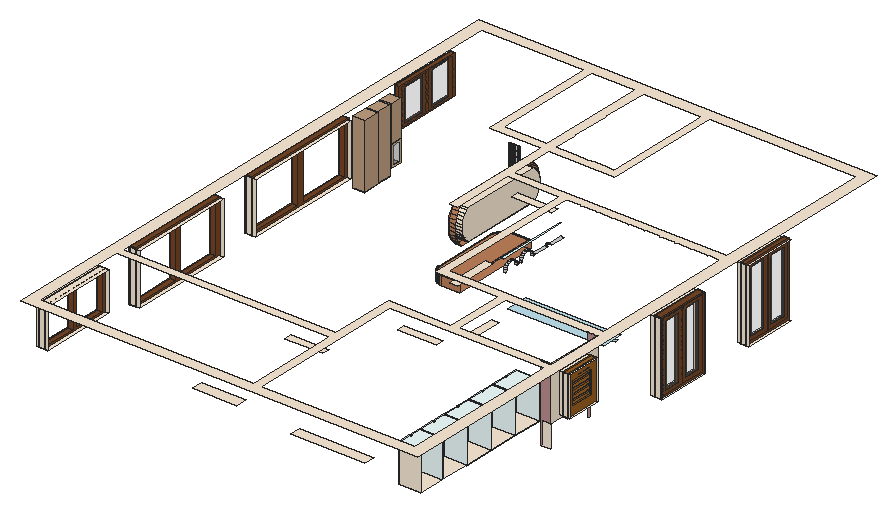
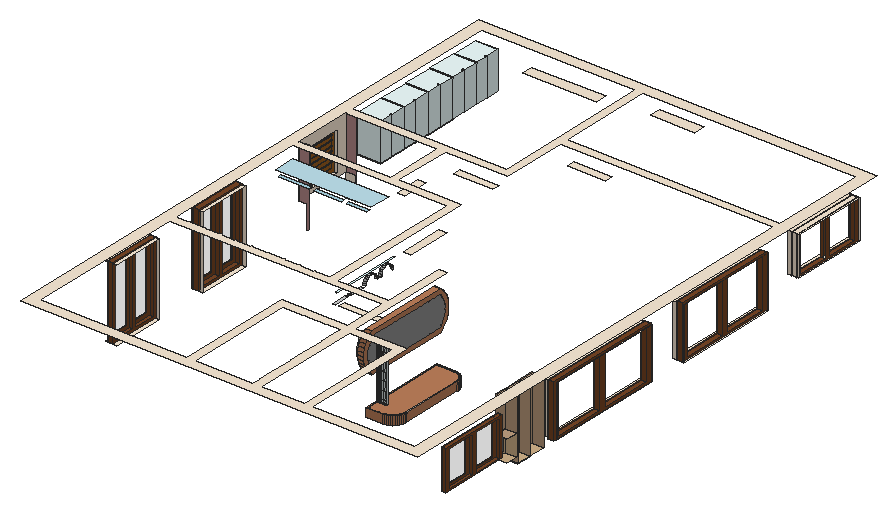
# SketchUp Ruby script. Lengths in inches.
U = 1.inch
M = Sketchup.active_model
def pt(a) = Geom::Point3d.new(a.map { |v| v * U })
def face(e, loops, mat)
  f = e.add_face(loops[0].map { |a| pt(a) })
  loops[1..].each { |l| e.add_face(l.map { |a| pt(a) }).erase! }
  f.material = f.back_material = mat if mat
  f
end
# faces: each face lists its corners as indices into pts; further lists are holes
def faces(e, pts, list, mat = nil) = list.each { |f| face(e, (f[0].is_a?(Array) ? f : [f]).map { |l| l.map { |i| pts[i] } }, mat) }
# xy, xz, yz: faces in a plane at the given z, y or x. An outline is a flat list of corners, or four numbers for a rectangle; further outlines are holes
def ring(l) = l.size == 4 ? [[l[0], l[1]], [l[2], l[1]], [l[2], l[3]], [l[0], l[3]]] : l.each_slice(2).to_a
def flat(e, list, mat, &to3) = list.each { |f| face(e, (f[0].is_a?(Array) ? f : [f]).map { |l| ring(l).map { |u, v| to3.(u, v) } }, mat) }
def xy(e, z, list, mat = nil) = flat(e, list, mat) { |x, y| [x, y, z] }
def xz(e, y, list, mat = nil) = flat(e, list, mat) { |x, z| [x, y, z] }
def yz(e, x, list, mat = nil) = flat(e, list, mat) { |y, z| [x, y, z] }
def lines(e, pts, list) = list.each { |a, b| e.add_line(pt(pts[a]), pt(pts[b])) }
# prism: a flat outline (further loops are holes) pulled along v
def prism(e, loops, v, mat = nil)
  f = face(e, loops, mat); d = Geom::Vector3d.new(v.map { |x| x * U })
  f.pushpull(f.normal.samedirection?(d) ? d.length : -d.length)
end
def box(e, o, s, mat = nil) = prism(e, [[o, [o[0] + s[0], o[1], o[2]], [o[0] + s[0], o[1] + s[1], o[2]], [o[0], o[1] + s[1], o[2]]]], [0, 0, s[2]], mat)
def at(x, y, z, deg = 0) = Geom::Transformation.translation(pt([x, y, z])) * Geom::Transformation.rotation(ORIGIN, Z_AXIS, deg.degrees)
def axes(o, x, y, z) = Geom::Transformation.new([*x, 0, *y, 0, *z, 0, *pt(o).to_a, 1])
def part(name) = M.definitions.add(name)
# library, detail: a bought-in or finely detailed component or shape, given as its bounding box
def library(name, o, s) = part(name).tap { |d| box(d.entities, o, s) }
def detail(e, o, s) = box(e.add_group.entities, o, s)
def put(e, d, t, mat = nil) = e.add_instance(d, t).tap { |i| i.material = mat if mat }
def group(e, t, mat = nil) = e.add_group.tap { |g| g.transformation = t; g.material = mat if mat }.entities
root = M.entities
M.materials.add("Plywood A 50cm\#1").color = [191, 159, 129]
M.materials.add("Wood EXN").color = [155, 95, 32]
M.materials.add("[0028_AntiqueWhite]").color = [250, 235, 215]
M.materials.add("[0035_Tan]").color = [210, 180, 140]
M.materials.add("[0090_LightCyan]").color = [224, 255, 255]
M.materials.add("[0092_Azure]").color = [240, 255, 255]
M.materials.add("[0095_LightBlue]").color = [173, 216, 230]
M.materials.add("[0100_SteelBlue]").color = [70, 130, 180]
M.materials.add("[0119_RosyBrown]").color = [188, 143, 143]
M.materials.add("[Carrera Marble]").color = [207, 207, 207]
M.materials.add("[Color M04]").color = [142, 142, 142]
M.materials.add("[Steel]").color = [192, 228, 240]
M.materials.add("[Translucent Glass Gray]").color = [128, 128, 128]
M.materials["[Translucent Glass Gray]"].alpha = 0.5
M.materials.add("[Translucent Glass Gray]1").color = [132, 132, 132]
M.materials["[Translucent Glass Gray]1"].alpha = 0.25
M.materials.add("[Wallpaper Dog Bone]").color = [213, 224, 224]
M.materials.add("[Wood Veneer 01]").color = [120, 70, 37]
M.materials.add("[Wood Veneer 02]").color = [190, 128, 91]
c1 = part("Group\#38")
prism(c1.entities,[[[0,1.97,1.57],[0,0.24,0.19],[0,0.22,0.17],[0,0.2,0.14],[0,0.19,0.11],[0,0.2,0.08],[0,0.2,0.05],[0,0.22,0.02],[0,0.24,0],[0,0.27,-0.02],[0,0.3,-0.03],[0,0.34,-0.03],[0,0.37,-0.02],[0,0.39,0],[0,2.36,1.57]]],[-67.04,0,0])
c2 = part("Wood+Window")
g1 = group(c2.entities,at(47.24,0,19.69),"Wood EXN")
g2 = group(g1,at(-47.24,5.91,0))
xy(g2,-19.69,[[0,-5.91,27.56,0]])
xy(g2,-17.72,[[1.97,-3.9375,25.59,0]])
xy(g2,-15.75,[[3.9375,-5.91,23.62,-4.92],[3.9375,-4.92,23.62,-3.9375]])
xy(g2,-3.9375,[[3.9375,-5.91,23.62,-4.92],[3.9375,-4.92,23.62,-3.9375]])
xy(g2,-1.97,[[1.97,-3.9375,25.59,0]])
xy(g2,0,[[0,-5.91,27.56,0]])
xz(g2,-5.91,[[[0,-19.69,27.56,0],[3.9375,-15.75,23.62,-3.9375]]])
xz(g2,-3.9375,[[[1.97,-17.72,25.59,-1.97],[3.9375,-15.75,23.62,-3.9375]]])
xz(g2,0,[[[0,-19.69,27.56,0],[1.97,-17.72,25.59,-1.97]]])
yz(g2,0,[[-5.91,-19.69,0,0]])
yz(g2,1.97,[[-3.9375,-17.72,0,-1.97]])
yz(g2,3.9375,[[-5.91,-15.75,-4.92,-3.9375],[-4.92,-15.75,-3.9375,-3.9375]])
yz(g2,23.62,[[-5.91,-15.75,-4.92,-3.9375],[-4.92,-15.75,-3.9375,-3.9375]])
yz(g2,25.59,[[-3.9375,-17.72,0,-1.97]])
yz(g2,27.56,[[-5.91,-19.69,0,0]])
g3 = group(g1,at(-20.98,5.88,-0.4))
put(g3,c1,axes([-24.3,0,-14.09],[-0.35238,0,0],[0,0,-1.2344],[0,-1,0]))
put(g3,c1,axes([-24.3,0,-11.66],[-0.35238,0,0],[0,0,-1.2344],[0,-1,0]))
put(g3,c1,axes([-24.3,0,-9.23],[-0.35238,0,0],[0,0,-1.2344],[0,-1,0]))
put(g3,c1,axes([-24.3,0,-6.8],[-0.35238,0,0],[0,0,-1.2344],[0,-1,0]))
put(g3,c1,axes([-24.3,0,-4.375],[-0.35238,0,0],[0,0,-1.2344],[0,-1,0]))
put(g3,c1,axes([-24.3,0,-1.94],[-0.35238,0,0],[0,0,-1.2344],[0,-1,0]))
c3 = part("Group\#31")
xy(c3.entities,0,[[0,0,19.69,1.18]],"[Wood Veneer 01]")
xy(c3.entities,2.76,[[2.76,0,16.93,1.18]],"[Wood Veneer 01]")
xy(c3.entities,60.24,[[2.76,0,16.93,1.18]],"[Wood Veneer 01]")
xy(c3.entities,62.99,[[0,0,19.69,1.18]],"[Wood Veneer 01]")
xz(c3.entities,0,[[2.76,2.76,16.93,60.24]],"[Translucent Glass Gray]1")
xz(c3.entities,0,[[[0,0,19.69,62.99],[2.76,2.76,16.93,60.24]]],"[Wood Veneer 01]")
xz(c3.entities,1.18,[[[0,0,19.69,62.99],[2.76,2.76,16.93,60.24]]],"[Wood Veneer 01]")
yz(c3.entities,0,[[0,0,1.18,62.99]],"[Wood Veneer 01]")
yz(c3.entities,2.76,[[0,2.76,1.18,60.24]],"[Wood Veneer 01]")
yz(c3.entities,16.93,[[0,2.76,1.18,60.24]],"[Wood Veneer 01]")
yz(c3.entities,19.69,[[0,0,1.18,62.99]],"[Wood Veneer 01]")
c4 = part("Group\#45")
prism(c4.entities,[[[0,0,66.93],[0,0,0],[45.28,0,0],[45.28,0,66.93]],[[43.31,0,1.97],[23.62,0,1.97],[23.62,0,64.96],[43.31,0,64.96]],[[21.65,0,64.96],[21.65,0,1.97],[1.97,0,1.97],[1.97,0,64.96]]],[0,5.91,0],"[Wood Veneer 01]")
c5 = part("pintu 2")
put(c5.entities,c3,axes([-252.08,-272.33,20.79],[0,0.96078,0],[-0.7,0,0],[0,0,0.89]))
put(c5.entities,c4,axes([-252.08,-295.03,19.04],[0,0.96078,0],[-0.7,0,0],[0,0,0.89]))
put(c5.entities,c3,axes([-252.08,-293.14,20.79],[0,0.96078,0],[-0.7,0,0],[0,0,0.89]))
put(c5.entities,c3,axes([-251.13,-360.52,20.79],[0,0.95802,0],[-0.861,0,0],[0,0,0.89]))
put(c5.entities,c4,axes([-251.13,-383.15,19.04],[0,0.95802,0],[-0.861,0,0],[0,0,0.89]))
put(c5.entities,c3,axes([-251.13,-381.27,20.79],[0,0.95802,0],[-0.861,0,0],[0,0,0.89]))
put(c5.entities,c3,axes([-569.23,-250.27,47.16],[0,1.26545,0],[-0.63714,0,0],[0,0,0.47766]))
put(c5.entities,c4,axes([-569.23,-252.76,46.22],[0,1.26545,0],[-0.63714,0,0],[0,0,0.47766]))
put(c5.entities,c3,axes([-569.23,-222.87,47.16],[0,1.26545,0],[-0.63714,0,0],[0,0,0.47766]))
g4 = group(c5.entities,at(-568.41,-522.34,36.16))
prism(g4,[[[0,0,42.82],[0,0,0],[0,85.875,0],[0,85.875,42.82]],[[0,82.14,1.26],[0,44.8,1.26],[0,44.8,41.56],[0,82.14,41.56]],[[0,41.07,41.56],[0,41.07,1.26],[0,3.73,1.26],[0,3.73,41.56]]],[-4.84,0,0],"[Wood Veneer 01]")
xy(g4,10.99,[[-4.61,-90.31,0,-63.41],[-4.61,-60.72,0,-33.82]],"[Wood Veneer 01]")
xz(g4,-90.31,[[-4.61,10.99,0,40.82]],"[Wood Veneer 01]")
xz(g4,-63.41,[[-4.61,10.99,0,40.82]],"[Wood Veneer 01]")
xz(g4,-33.82,[[-4.61,10.99,0,40.82]],"[Wood Veneer 01]")
yz(g4,-4.61,[[[-93,10.0625,-31.125,41.75],[-90.31,10.99,-63.41,40.82],[-60.72,10.99,-33.82,40.82]]],"[Wood Veneer 01]")
yz(g4,0,[[[-93,10.0625,-31.125,41.75],[-90.31,10.99,-63.41,40.82],[-60.72,10.99,-33.82,40.82]]],"[Wood Veneer 01]")
put(c5.entities,c4,axes([-568.41,-403.84,36.16],[0,2.18123,0],[-0.82,0,0],[0,0,0.63976]))
c6 = part("jendela")
put(c6.entities,c5,at(128.6,134.95,33.46))
xy(root,50.86,[[120.1875,279.625,118.875,279.71,117.58,279.97,116.34,280.39,115.16,280.97,114.0625,281.7,113.07,282.57,112.2,283.5625,111.47,284.66,110.89,285.84,110.47,287.08,110.21,288.375,110.125,289.6875,110.125,341.09,110.22,342.52,110.5,343.91,110.96,345.27,111.59,346.55,112.38,347.73,113.32,348.8,114.39,349.75,115.58,350.54,116.86,351.17,118.21,351.63,119.61,351.91,121.03,352,134.6875,352,134.6875,279.625]],"[Wood Veneer 02]")
xy(root,52.5,[[315,249.4375,324,292.8125],[315,337.5625,324,381.0625]],"[0028_AntiqueWhite]")
xy(root,57.73,[[[120.1875,279.625,134.6875,279.625,134.6875,352,121.03,352,119.61,351.91,118.21,351.63,116.86,351.17,115.58,350.54,114.39,349.75,113.32,348.8,112.38,347.73,111.59,346.55,110.96,345.27,110.5,343.91,110.22,342.52,110.125,341.09,110.125,289.6875,110.21,288.375,110.47,287.08,110.89,285.84,111.47,284.66,112.2,283.5625,113.07,282.57,114.0625,281.7,115.16,280.97,116.34,280.39,117.58,279.97,118.875,279.71],[120.1875,280.51,118.99,280.59,117.8125,280.83,116.68,281.21,115.6,281.74,114.6,282.41,113.7,283.2,112.91,284.1,112.24,285.1,111.71,286.18,111.33,287.3125,111.09,288.49,111.01,289.6875,111.01,341.09,111.1,342.4,111.35,343.68,111.78,344.93,112.36,346.1,113.08,347.19,113.95,348.18,114.93,349.04,116.02,349.77,117.2,350.35,118.44,350.77,119.73,351.03,121.03,351.11,133.8,351.11,133.8,280.51]]],"[Wood Veneer 02]")
xy(root,57.79,[[120.1875,280.51,133.8,280.51,133.8,351.11,121.03,351.11,119.73,351.03,118.44,350.77,117.2,350.35,116.02,349.77,114.93,349.04,113.95,348.18,113.08,347.19,112.36,346.1,111.78,344.93,111.35,343.68,111.1,342.4,111.01,341.09,111.01,289.6875,111.09,288.49,111.33,287.3125,111.71,286.18,112.24,285.1,112.91,284.1,113.7,283.2,114.6,282.41,115.6,281.74,116.68,281.21,117.8125,280.83,118.99,280.59]],"[Wood Veneer 02]")
xy(root,61.75,[[9,328.1875,18.125,341.8125],[9,342.3125,18.125,354.625]],"[0035_Tan]")
xy(root,62.3125,[[9,328.1875,18.125,341.8125],[9,342.3125,18.125,354.625]],"[0035_Tan]")
xy(root,67.4375,[[9,355.875,18.125,365.4375]],"[0035_Tan]")
xy(root,68.72,[[17.9375,357.15,18.125,364.16]],"[Translucent Glass Gray]")
xy(root,69.625,[[0,110.25,9,196.125],[0,228.75,9,325.9375]],"[0028_AntiqueWhite]")
xy(root,72.59,[[109.5,361.5625,110.04,361.9375],[110.125,361.5625,110.67,361.9375],[110.75,361.5625,111.3,361.9375],[111.38,361.5625,111.92,361.9375],[112.01,361.5625,112.55,361.9375],
  [112.63,361.5625,113.18,361.9375],[113.26,361.5625,113.8,361.9375],[113.89,361.5625,114.43,361.9375],[114.51,361.5625,115.06,361.9375],[115.14,361.5625,115.68,361.9375],
  [115.76,361.5625,116.31,361.9375],[116.39,361.5625,116.93,361.9375],[117.02,361.5625,117.5625,361.9375],[117.64,361.5625,118.1875,361.9375]],"[Wallpaper Dog Bone]")
xy(root,79.6875,[[0,17.25,9,79.125],[315,155.5625,324,184.3125]],"[0028_AntiqueWhite]")
xy(root,83.43,[[17.9375,357.15,18.125,364.16]],"[Translucent Glass Gray]")
xy(root,83.5625,[[296.5625,61.7,315,61.7,315,85.7,296.5625,85.7,296.5625,74.95,297.6875,74.95,297.6875,74.14,296.5625,74.14],[296.5625,86.4,315,86.4,315,110.4,296.5625,110.4,296.5625,100.15,297.8125,100.15,297.8125,99.4,296.5625,99.4],[296.5625,111,315,111,315,135,296.5625,135,296.5625,124.25,297.5,124.25,297.5,123.4375,296.5625,123.4375]],"[0092_Azure]")
xy(root,83.82,[[129.5,282.13,134.6875,352.45]],"[Wood Veneer 02]")
xy(root,84.26,[[296.5625,14.9375,296.5625,26,297.625,26,297.625,26.76,296.5625,26.76,296.5625,36.57,315,36.57,315,14.9375],[296.5625,37.07,296.5625,49.39,298.25,49.39,298.25,50.26,296.5625,50.26,296.5625,61.2,315,61.2,315,37.07],[296.5625,61.7,296.5625,74.14,298.0625,74.14,298.0625,74.95,296.5625,74.95,296.5625,85.7,315,85.7,315,61.7],[296.5625,86.4,296.5625,99.4,297.4375,99.4,297.4375,100.15,296.5625,100.15,296.5625,110.4,315,110.4,315,86.4],[296.5625,111,296.5625,123.4375,297.5,123.4375,297.5,124.25,296.5625,124.25,296.5625,135,315,135,315,111]],"[0028_AntiqueWhite]")
xy(root,84.71,[[9,355.875,18.125,365.4375]],"[0035_Tan]")
xy(root,85.02,[[9,355.875,18.125,365.4375]],"Plywood A 50cm\#1")
xy(root,87.49,[[129.5,283.61,138.1875,351.1]],"[0028_AntiqueWhite]")
xy(root,96.64,[[190.125,267.5625,191.3125,270.5625],[190.125,285.5,192.4375,297.5],[190.125,301.5,192.4375,313.5]],"[Carrera Marble]")
xy(root,100.49,[[221,0,280.875,9]],"[0028_AntiqueWhite]")
xy(root,105.32,[[240.3125,216.125,257.1875,218.875],[261.3125,216.125,283.9375,218.875],[287.9375,216.125,312.6875,218.875]],"[0095_LightBlue]")
xy(root,106,[[141,0,177,9],[146.25,87,177,93],[195.375,141,227.25,147],[234,167.4375,240,188.3],[183,209.4375,189,245.9375],
  [144,321,177,327]],"[0028_AntiqueWhite]")
xy(root,106,[[189,255.0625,190.125,313.875]],"[0090_LightCyan]")
xy(root,109.75,[[237,201,315,218.875]],"[Steel]")
xy(root,111.5,[[315,155.5625,324,184.3125],[315,249.4375,324,292.8125],[315,337.5625,324,381.0625]],"[0028_AntiqueWhite]")
xy(root,111.66,[[0,17.25,9,79.125],[0,110.25,9,196.125],[0,228.75,9,325.9375]],"[0028_AntiqueWhite]")
xy(root,112.03,[[129.5,283.61,138.1875,351.1]],"[0028_AntiqueWhite]")
xy(root,114.3125,[[9,328.1875,18.125,341.8125],[9,342.3125,18.125,354.625],[9,355.875,18.125,365.4375]],"Plywood A 50cm\#1")
xy(root,114.75,[[296.5625,14.9375,315,14.9375,315,36.57,296.5625,36.57,296.5625,26.76,297.625,26.76,297.625,26,296.5625,26],[296.5625,37.07,315,37.07,315,61.2,296.5625,61.2,296.5625,50.26,298.25,50.26,298.25,49.39,296.5625,49.39],[296.5625,61.7,315,61.7,315,85.7,296.5625,85.7,296.5625,74.95,298.0625,74.95,298.0625,74.14,296.5625,74.14],[296.5625,86.4,315,86.4,315,110.4,296.5625,110.4,296.5625,100.15,297.4375,100.15,297.4375,99.4,296.5625,99.4],[296.5625,111,315,111,315,135,296.5625,135,296.5625,124.25,297.5,124.25,297.5,123.4375,296.5625,123.4375]],"[0092_Azure]")
xy(root,115.7,[[129.5,282.13,134.6875,352.45]],"[Wood Veneer 02]")
xy(root,120,[[[0,0,324,468],[9,93,9,459,93,459,93,363,134.6875,363,134.6875,270,141,270,141,321,183,321,183,195,234,195,234,147,183,147,183,93],[141,327,141,363,195,363,195,459,315,459,315,327],[189,9,315,141],[189,201,189,320.25,190.25,320.25,190.25,321,201,321,201,320.25,201.9,320.25,201.9,321,213.9,321,213.9,320.25,214.8,320.25,214.8,321,226.8,321,226.8,320.25,227.7,320.25,227.7,321,239.7,321,239.7,320.25,240.625,320.25,240.625,321,252.65,321,252.65,320.25,253.5,320.25,253.5,321,265.51,321,265.51,320.25,266.47,320.25,266.47,321,278.4,321,278.4,320,279.3,320,279.3,321,291.36,321,291.36,320.4375,292.2,320.4375,292.2,321,304.2,321,304.2,320.375,305.01,320.375,305.01,321,314.1875,321,314.1875,320.375,315,320.375,315,201],[9,9,183,87],[141,369,141,370,141.1875,370,141.1875,373,141,373,141,373.43,141.1875,373.43,141.1875,385.37,141,385.37,141,385.8,141.1875,385.8,141.1875,388.8,141,388.8,141,389.21,141.1875,389.21,141.1875,401.2,141,401.2,141,401.6,141.1875,401.6,141.1875,404.63,141,404.63,141,405,141.1875,405,141.1875,417,141,417,141,417.42,141.1875,417.42,141.1875,420.4,141,420.4,141,420.8,141.1875,420.8,141.1875,432.8,141,432.8,141,433.18,141.1875,433.18,141.1875,436.19,141,436.19,141,436.6,141.1875,436.6,141.1875,448.6,141,448.6,141,449,141.1875,449,141.1875,452,141,452,141,452.4,141.1875,452.4,141.1875,459,189,459,189,369,188,369,188,369.25,185,369.25,185,369,184.47,369,184.47,369.25,172.49,369.25,172.49,369,172.1,369,172.1,369.25,169.1,369.25,169.1,369,168.7,369,168.7,369.25,156.7,369.25,156.7,369,156.2,369,156.2,369.25,153.14,369.25,153.14,369,152.78,369,152.78,369.25,142.02,369.25,142.02,369],[240,147,315,195],[99,369,134.6875,459]]],"[0028_AntiqueWhite]")
xz(root,14.9375,[[296.5625,84.26,315,114.75]],"[0028_AntiqueWhite]")
xz(root,17.25,[[0,79.6875,9,111.66]],"[0028_AntiqueWhite]")
xz(root,26,[[296.5625,84.26,297.625,114.75]],"[0100_SteelBlue]")
xz(root,26.76,[[296.5625,84.26,297.625,114.75]],"[0100_SteelBlue]")
xz(root,36.57,[[296.5625,84.26,315,114.75]],"[0092_Azure]")
xz(root,37.07,[[296.5625,84.26,315,114.75]],"[0092_Azure]")
xz(root,49.39,[[296.5625,84.26,298.25,114.75]],"[0100_SteelBlue]")
xz(root,50.26,[[296.5625,84.26,298.25,114.75]],"[0100_SteelBlue]")
xz(root,61.2,[[296.5625,84.26,315,114.75]],"[0092_Azure]")
xz(root,61.7,[[296.5625,84.26,315,114.75]],"[0092_Azure]")
xz(root,74.14,[[296.5625,84.26,298.0625,114.75]],"[0100_SteelBlue]")
xz(root,74.95,[[296.5625,84.26,298.0625,114.75]],"[0100_SteelBlue]")
xz(root,79.125,[[0,79.6875,9,111.66]],"[0028_AntiqueWhite]")
xz(root,85.7,[[296.5625,84.26,315,114.75]],"[0092_Azure]")
xz(root,86.4,[[296.5625,84.26,315,114.75]],"[0092_Azure]")
xz(root,99.4,[[296.5625,84.26,297.4375,114.75]],"[0100_SteelBlue]")
xz(root,100.15,[[296.5625,84.26,297.4375,114.75]],"[0100_SteelBlue]")
xz(root,110.25,[[0,69.625,9,111.66]],"[0028_AntiqueWhite]")
xz(root,110.4,[[296.5625,84.26,315,114.75]],"[0092_Azure]")
xz(root,111,[[296.5625,84.26,315,114.75]],"[0092_Azure]")
xz(root,123.4375,[[296.5625,84.26,297.5,114.75]],"[0100_SteelBlue]")
xz(root,124.25,[[296.5625,84.26,297.5,114.75]],"[0100_SteelBlue]")
xz(root,135,[[296.5625,84.26,315,114.75]],"[0092_Azure]")
xz(root,147,[[308.25,58,315,76.6875]],"[0028_AntiqueWhite]")
xz(root,147,[[306.6875,58,306.6875,120,315,120,315,76.6875,308.25,76.6875,308.25,58]],"[0119_RosyBrown]")
xz(root,155.5625,[[315,79.6875,324,111.5]],"[0028_AntiqueWhite]")
xz(root,184.3125,[[315,79.6875,324,111.5]],"[0028_AntiqueWhite]")
xz(root,195,[[307.3125,58.08,308.25,58.08,308.25,76.6875,315,76.6875,315,120,307.3125,120]],"[0119_RosyBrown]")
xz(root,196.125,[[0,69.625,9,111.66]],"[0028_AntiqueWhite]")
xz(root,228.75,[[0,69.625,9,111.66]],"[0028_AntiqueWhite]")
xz(root,249.4375,[[315,52.5,324,111.5]],"[0028_AntiqueWhite]")
xz(root,279.625,[[120.1875,50.86,134.6875,57.73]],"[Wood Veneer 02]")
xz(root,280.51,[[120.1875,57.73,133.8,57.79]],"[0028_AntiqueWhite]")
xz(root,292.8125,[[315,52.5,324,111.5]],"[0028_AntiqueWhite]")
xz(root,325.9375,[[0,69.625,9,111.66]],"[0028_AntiqueWhite]")
xz(root,328.1875,[[9,62.3125,18.125,114.3125]],"Plywood A 50cm\#1")
xz(root,337.5625,[[315,52.5,324,111.5]],"[0028_AntiqueWhite]")
xz(root,341.8125,[[9,62.3125,18.125,114.3125]],"[0035_Tan]")
xz(root,342.3125,[[9,62.3125,18.125,114.3125]],"Plywood A 50cm\#1")
xz(root,351.11,[[121.03,57.73,133.8,57.79]],"[0028_AntiqueWhite]")
xz(root,352,[[121.03,50.86,134.6875,57.73]],"[Wood Veneer 02]")
xz(root,354.625,[[9,62.3125,18.125,114.3125]],"Plywood A 50cm\#1")
xz(root,355.875,[[9,85.02,18.125,114.3125]],"Plywood A 50cm\#1")
xz(root,355.875,[[9,67.4375,18.125,84.71]],"[0035_Tan]")
xz(root,357.15,[[17.9375,68.72,18.125,83.43]],"[0028_AntiqueWhite]")
xz(root,361.5625,[[109.5,73.1875,109.82,115.7],[110.02,73.1875,110.35,115.7],[110.55,73.1875,110.87,115.7],[111.07,73.1875,111.39,115.7],[111.59,73.1875,111.92,115.7],
  [112.12,73.1875,112.44,115.7],[112.64,73.1875,112.96,115.7],[113.16,73.1875,113.49,115.7],[113.6875,73.1875,114.01,115.7],[114.21,73.1875,114.54,115.7],
  [114.73,73.1875,115.06,115.7],[115.26,73.1875,115.58,115.7],[115.78,73.1875,116.11,115.7],[116.3,73.1875,116.63,115.7],[116.83,73.1875,117.15,115.7],
  [117.35,73.1875,117.68,115.7],[117.875,73.1875,118.2,115.7]],"[Wallpaper Dog Bone]")
yz(root,17.9375,[[357.15,68.72,364.16,83.43]],"[Translucent Glass Gray]")
yz(root,18.125,[[328.1875,62.3125,341.8125,114.3125],[342.3125,62.3125,354.625,114.3125],[355.875,85.02,365.4375,114.3125]],"Plywood A 50cm\#1")
yz(root,18.125,[[[355.875,67.4375,365.4375,84.71],[357.15,68.72,364.16,83.43]]],"[0035_Tan]")
yz(root,109.5,[[361.5625,73.1875,361.9375,115.7]],"[Wallpaper Dog Bone]")
yz(root,110.125,[[289.6875,50.86,341.09,57.73]],"[Wood Veneer 02]")
yz(root,111.01,[[289.6875,57.73,341.09,57.79]],"[0028_AntiqueWhite]")
yz(root,129.5,[[283.61,87.49,282.68,88.38,281.15,90.35,279.93,92.52,279.04,94.85,278.5,97.28,278.3125,99.76,278.5,102.24,279.04,104.67,279.93,107,281.15,109.17,282.68,111.14,283.61,112.03,351.1,112.03,352.2,111.09,353.83,109.17,355.15,107.03,356.11,104.71,356.7,102.27,356.89,99.76,356.7,97.25,356.11,94.81,355.15,92.49,353.83,90.35,352.2,88.43,351.1,87.49]],"[Color M04]")
yz(root,129.5,[[[282.13,83.82,279.94,85.92,278.09,88.3125,276.6,90.95,275.51,93.78,274.85,96.74,274.63,99.76,274.85,102.78,275.51,105.74,276.6,108.57,278.09,111.21,279.94,113.6,282.13,115.7,352.45,115.7,354.8,113.69,356.8125,111.34,358.43,108.7,359.61,105.85,360.33,102.84,360.58,99.76,360.33,96.68,359.61,93.67,358.43,90.82,356.8125,88.18,354.8,85.83,352.45,83.82],[283.61,87.49,351.1,87.49,352.2,88.43,353.83,90.35,355.15,92.49,356.11,94.81,356.7,97.25,356.89,99.76,356.7,102.27,356.11,104.71,355.15,107.03,353.83,109.17,352.2,111.09,351.1,112.03,283.61,112.03,282.68,111.14,281.15,109.17,279.93,107,279.04,104.67,278.5,102.24,278.3125,99.76,278.5,97.28,279.04,94.85,279.93,92.52,281.15,90.35,282.68,88.38]]],"[Wood Veneer 02]")
yz(root,133.8,[[280.51,57.73,351.11,57.79]],"[0028_AntiqueWhite]")
yz(root,138.1875,[[283.61,87.49,282.68,88.38,281.15,90.35,279.93,92.52,279.04,94.85,278.5,97.28,278.3125,99.76,278.5,102.24,279.04,104.67,279.93,107,281.15,109.17,282.68,111.14,283.61,112.03,351.1,112.03,352.2,111.09,353.83,109.17,355.15,107.03,356.11,104.71,356.7,102.27,356.89,99.76,356.7,97.25,356.11,94.81,355.15,92.49,353.83,90.35,352.2,88.43,351.1,87.49]],"[0028_AntiqueWhite]")
yz(root,296.5625,[[14.9375,84.26,26,114.75],[26.76,84.26,36.57,114.75],[37.07,84.26,49.39,114.75],[50.26,84.26,61.2,114.75],[61.7,84.26,74.14,114.75],
  [74.95,84.26,85.7,114.75],[86.4,84.26,99.4,114.75],[100.15,84.26,110.4,114.75],[111,84.26,123.4375,114.75],[124.25,84.26,135,114.75]],"[0092_Azure]")
yz(root,297.4375,[[99.4,84.26,100.15,114.75]],"[0100_SteelBlue]")
yz(root,297.5,[[123.4375,84.26,124.25,114.75]],"[0100_SteelBlue]")
yz(root,297.625,[[26,84.26,26.76,114.75]],"[0100_SteelBlue]")
yz(root,298.0625,[[74.14,84.26,74.95,114.75]],"[0100_SteelBlue]")
yz(root,298.25,[[49.39,84.26,50.26,114.75]],"[0100_SteelBlue]")
yz(root,315,[[[147,76.6875,195,120],[155.5625,79.6875,184.3125,111.5]]],"[0028_AntiqueWhite]")
p = [[120.1875,279.625,50.86],[120.1875,279.625,57.73],[118.875,279.71,57.73],[118.875,279.71,50.86],[117.58,279.97,57.73],[117.58,279.97,50.86],
  [116.34,280.39,57.73],[116.34,280.39,50.86],[115.16,280.97,57.73],[115.16,280.97,50.86],[114.0625,281.7,57.73],[114.0625,281.7,50.86],
  [113.07,282.57,57.73],[113.07,282.57,50.86],[112.2,283.5625,57.73],[112.2,283.5625,50.86],[111.47,284.66,57.73],[111.47,284.66,50.86],
  [110.89,285.84,57.73],[110.89,285.84,50.86],[110.47,287.08,57.73],[110.47,287.08,50.86],[110.21,288.375,57.73],[110.21,288.375,50.86],
  [110.125,289.6875,57.73],[110.125,289.6875,50.86],[110.125,341.09,50.86],[110.125,341.09,57.73],[110.22,342.52,57.73],[110.22,342.52,50.86],
  [110.5,343.91,57.73],[110.5,343.91,50.86],[110.96,345.27,57.73],[110.96,345.27,50.86],[111.59,346.55,57.73],[111.59,346.55,50.86],
  [112.38,347.73,57.73],[112.38,347.73,50.86],[113.32,348.8,57.73],[113.32,348.8,50.86],[114.39,349.75,57.73],[114.39,349.75,50.86],
  [115.58,350.54,57.73],[115.58,350.54,50.86],[116.86,351.17,57.73],[116.86,351.17,50.86],[118.21,351.63,57.73],[118.21,351.63,50.86],
  [119.61,351.91,57.73],[119.61,351.91,50.86],[121.03,352,57.73],[121.03,352,50.86],[120.1875,280.51,57.79],[118.99,280.59,57.79],
  [118.99,280.59,57.73],[120.1875,280.51,57.73],[117.8125,280.83,57.79],[117.8125,280.83,57.73],[116.68,281.21,57.79],[116.68,281.21,57.73],
  [115.6,281.74,57.79],[115.6,281.74,57.73],[114.6,282.41,57.79],[114.6,282.41,57.73],[113.7,283.2,57.79],[113.7,283.2,57.73],
  [112.91,284.1,57.79],[112.91,284.1,57.73],[112.24,285.1,57.79],[112.24,285.1,57.73],[111.71,286.18,57.79],[111.71,286.18,57.73],
  [111.33,287.3125,57.79],[111.33,287.3125,57.73],[111.09,288.49,57.79],[111.09,288.49,57.73],[111.01,289.6875,57.79],[111.01,289.6875,57.73],
  [111.01,341.09,57.79],[111.1,342.4,57.79],[111.1,342.4,57.73],[111.01,341.09,57.73],[111.35,343.68,57.79],[111.35,343.68,57.73],
  [111.78,344.93,57.79],[111.78,344.93,57.73],[112.36,346.1,57.79],[112.36,346.1,57.73],[113.08,347.19,57.79],[113.08,347.19,57.73],
  [113.95,348.18,57.79],[113.95,348.18,57.73],[114.93,349.04,57.79],[114.93,349.04,57.73],[116.02,349.77,57.79],[116.02,349.77,57.73],
  [117.2,350.35,57.79],[117.2,350.35,57.73],[118.44,350.77,57.79],[118.44,350.77,57.73],[119.73,351.03,57.79],[119.73,351.03,57.73],
  [121.03,351.11,57.79],[121.03,351.11,57.73],[134.6875,282.13,83.82],[134.6875,279.94,85.92],[129.5,279.94,85.92],[129.5,282.13,83.82],
  [134.6875,354.8,85.83],[134.6875,352.45,83.82],[129.5,352.45,83.82],[129.5,354.8,85.83],[134.6875,356.8125,88.18],[129.5,356.8125,88.18],
  [134.6875,278.09,88.3125],[129.5,278.09,88.3125],[129.5,283.61,87.49],[129.5,282.68,88.38],[138.1875,282.68,88.38],[138.1875,283.61,87.49],
  [129.5,352.2,88.43],[129.5,351.1,87.49],[138.1875,351.1,87.49],[138.1875,352.2,88.43],[134.6875,358.43,90.82],[129.5,358.43,90.82],
  [134.6875,276.6,90.95],[129.5,276.6,90.95],[129.5,281.15,90.35],[138.1875,281.15,90.35],[129.5,353.83,90.35],[138.1875,353.83,90.35],
  [129.5,355.15,92.49],[138.1875,355.15,92.49],[129.5,279.93,92.52],[138.1875,279.93,92.52],[134.6875,359.61,93.67],[129.5,359.61,93.67],
  [134.6875,275.51,93.78],[129.5,275.51,93.78],[129.5,279.04,94.85],[138.1875,279.04,94.85],[129.5,356.11,94.81],[138.1875,356.11,94.81],
  [134.6875,360.33,96.68],[129.5,360.33,96.68],[134.6875,274.85,96.74],[129.5,274.85,96.74],[129.5,278.5,97.28],[138.1875,278.5,97.28],
  [129.5,356.7,97.25],[138.1875,356.7,97.25],[190.125,255.27,98.2],[190.125,255.0625,96.64],[192.4375,255.0625,96.64],[192.4375,255.27,98.2],
  [190.125,267.0625,96.64],[190.125,266.86,98.2],[192.4375,266.86,98.2],[192.4375,267.0625,96.64],[190.125,271.27,98.2],[190.125,271.0625,96.64],
  [192.4375,271.0625,96.64],[192.4375,271.27,98.2],[190.125,283.0625,96.64],[190.125,282.86,98.2],[192.4375,282.86,98.2],[192.4375,283.0625,96.64],
  [190.125,298.05,97.03],[190.125,298,96.64],[191,298,96.64],[191,298.05,97.03],[190.125,301,96.64],[190.125,300.95,97.03],
  [191,300.95,97.03],[191,301,96.64],[134.6875,274.63,99.76],[129.5,274.63,99.76],[134.6875,360.58,99.76],[129.5,360.58,99.76],
  [190.125,298.2,97.39],[191,298.2,97.39],[190.125,300.8,97.39],[191,300.8,97.39],[129.5,278.3125,99.76],[138.1875,278.3125,99.76],
  [129.5,356.89,99.76],[138.1875,356.89,99.76],[190.125,298.4375,97.7],[191,298.4375,97.7],[190.125,300.5625,97.7],[191,300.5625,97.7],
  [190.125,298.75,97.94],[191,298.75,97.94],[190.125,300.25,97.94],[191,300.25,97.94],[190.125,299.11,98.09],[191,299.11,98.09],
  [190.125,299.89,98.09],[191,299.89,98.09],[190.125,299.5,98.14],[191,299.5,98.14],[190.125,255.87,99.64],[192.4375,255.87,99.64],
  [190.125,266.26,99.64],[192.4375,266.26,99.64],[190.125,271.87,99.64],[192.4375,271.87,99.64],[190.125,282.26,99.64],[192.4375,282.26,99.64],
  [190.125,256.82,100.89],[192.4375,256.82,100.89],[190.125,265.31,100.89],[192.4375,265.31,100.89],[190.125,272.82,100.89],[192.4375,272.82,100.89],
  [190.125,281.31,100.89],[192.4375,281.31,100.89],[134.6875,274.85,102.78],[129.5,274.85,102.78],[129.5,278.5,102.24],[138.1875,278.5,102.24],
  [129.5,356.7,102.27],[138.1875,356.7,102.27],[134.6875,360.33,102.84],[129.5,360.33,102.84],[190.125,258.0625,101.84],[192.4375,258.0625,101.84],
  [190.125,264.0625,101.84],[192.4375,264.0625,101.84],[190.125,274.0625,101.84],[192.4375,274.0625,101.84],[190.125,280.0625,101.84],[192.4375,280.0625,101.84],
  [190.125,259.51,102.4375],[192.4375,259.51,102.4375],[190.125,262.62,102.4375],[192.4375,262.62,102.4375],[190.125,275.51,102.4375],[192.4375,275.51,102.4375],
  [190.125,278.62,102.4375],[192.4375,278.62,102.4375],[129.5,279.04,104.67],[138.1875,279.04,104.67],[129.5,356.11,104.71],[138.1875,356.11,104.71],
  [190.125,261.0625,102.64],[192.4375,261.0625,102.64],[190.125,277.0625,102.64],[192.4375,277.0625,102.64],[134.6875,275.51,105.74],[129.5,275.51,105.74],
  [134.6875,359.61,105.85],[129.5,359.61,105.85],[129.5,279.93,107],[138.1875,279.93,107],[129.5,355.15,107.03],[138.1875,355.15,107.03],
  [134.6875,276.6,108.57],[129.5,276.6,108.57],[134.6875,358.43,108.7],[129.5,358.43,108.7],[129.5,281.15,109.17],[138.1875,281.15,109.17],
  [129.5,353.83,109.17],[138.1875,353.83,109.17],[134.6875,278.09,111.21],[129.5,278.09,111.21],[134.6875,356.8125,111.34],[129.5,356.8125,111.34],
  [129.5,282.68,111.14],[138.1875,282.68,111.14],[129.5,352.2,111.09],[138.1875,352.2,111.09],[129.5,283.61,112.03],[138.1875,283.61,112.03],
  [129.5,351.1,112.03],[138.1875,351.1,112.03],[134.6875,279.94,113.6],[129.5,279.94,113.6],[134.6875,354.8,113.69],[129.5,354.8,113.69],
  [134.6875,282.13,115.7],[129.5,282.13,115.7],[134.6875,352.45,115.7],[129.5,352.45,115.7]]
faces(root,p,[[0,1,2,3],[3,2,4,5],[5,4,6,7],[7,6,8,9],[9,8,10,11],[11,10,12,13],[13,12,14,15],[15,14,16,17],
  [17,16,18,19],[19,18,20,21],[21,20,22,23],[23,22,24,25],[26,27,28,29],[29,28,30,31],[31,30,32,33],[33,32,34,35],
  [35,34,36,37],[37,36,38,39],[39,38,40,41],[41,40,42,43],[43,42,44,45],[45,44,46,47],[47,46,48,49],[49,48,50,51],
  [104,105,106,107],[108,109,110,111],[112,108,111,113],[105,114,115,106],[124,112,113,125],[114,126,127,115],[136,124,125,137],[126,138,139,127],
  [144,136,137,145],[138,146,147,139],[146,176,177,147],[178,144,145,179],[176,218,219,177],[224,178,179,225],[218,250,251,219],[252,224,225,253],
  [250,258,259,251],[260,252,253,261],[258,266,267,259],[268,260,261,269],[266,278,279,267],[280,268,269,281],[278,282,283,279],[284,280,281,285]],"[Wood Veneer 02]")
faces(root,p,[[52,53,54,55],[53,56,57,54],[56,58,59,57],[58,60,61,59],[60,62,63,61],[62,64,65,63],[64,66,67,65],[66,68,69,67],
  [68,70,71,69],[70,72,73,71],[72,74,75,73],[74,76,77,75],[78,79,80,81],[79,82,83,80],[82,84,85,83],[84,86,87,85],
  [86,88,89,87],[88,90,91,89],[90,92,93,91],[92,94,95,93],[94,96,97,95],[96,98,99,97],[98,100,101,99],[100,102,103,101],
  [116,117,118,119],[120,121,122,123],[117,128,129,118],[130,120,123,131],[132,130,131,133],[128,134,135,129],[134,140,141,135],[142,132,133,143],
  [140,148,149,141],[150,142,143,151],[148,184,185,149],[186,150,151,187],[184,220,221,185],[222,186,187,223],[220,242,243,221],[244,222,223,245],
  [242,254,255,243],[256,244,245,257],[254,262,263,255],[264,256,257,265],[262,270,271,263],[272,264,265,273],[270,274,275,271],[276,272,273,277]],"[0028_AntiqueWhite]")
faces(root,p,[[152,153,154,155],[156,157,158,159],[160,161,162,163],[164,165,166,167],[168,169,170,171],[172,173,174,175],[180,168,171,181],[173,182,183,174],
  [188,180,181,189],[182,190,191,183],[192,188,189,193],[190,194,195,191],[196,192,193,197],[194,198,199,195],[200,196,197,201],[198,200,201,199],
  [202,152,155,203],[157,204,205,158],[206,160,163,207],[165,208,209,166],[210,202,203,211],[204,212,213,205],[214,206,207,215],[208,216,217,209],
  [226,210,211,227],[212,228,229,213],[230,214,215,231],[216,232,233,217],[234,226,227,235],[228,236,237,229],[238,230,231,239],[232,240,241,233],
  [246,234,235,247],[236,246,247,237],[248,238,239,249],[240,248,249,241]],"[Carrera Marble]")
put(root,c2,axes([322.17,155.5625,79.09],[0,1.04321,0],[-0.69,0,0],[0,0,1.6463]))
put(root,c6,at(445.72,497.65,0))
